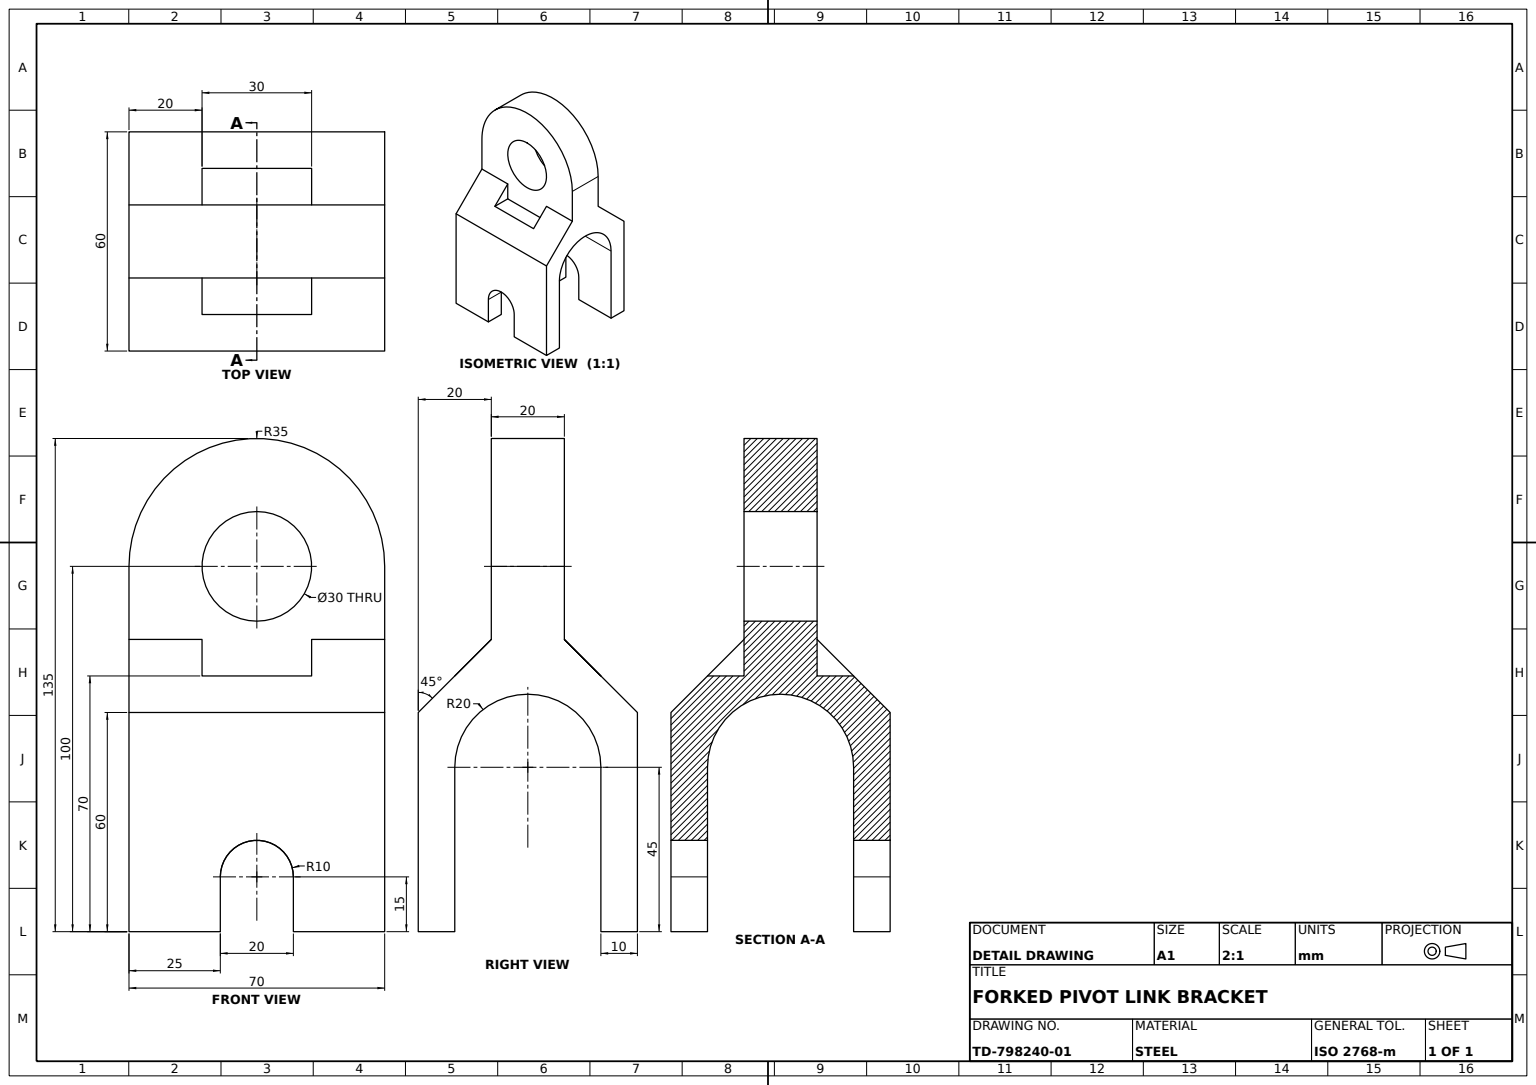
ISO-10303-21;
HEADER;
FILE_DESCRIPTION((''),'2;1');
FILE_NAME('','',(''),(''),'','','');
FILE_SCHEMA(('AUTOMOTIVE_DESIGN'));
ENDSEC;
DATA;
#1=APPLICATION_CONTEXT('');
#2=PRODUCT_CONTEXT('',#1,'mechanical');
#3=PRODUCT('','','',(#2));
#4=PRODUCT_DEFINITION_FORMATION('','',#3);
#5=PRODUCT_DEFINITION_CONTEXT('',#1,'design');
#6=PRODUCT_DEFINITION('','',#4,#5);
#7=PRODUCT_DEFINITION_SHAPE('','',#6);
#8=(LENGTH_UNIT()NAMED_UNIT(*)SI_UNIT(.MILLI.,.METRE.));
#9=(NAMED_UNIT(*)PLANE_ANGLE_UNIT()SI_UNIT($,.RADIAN.));
#10=(NAMED_UNIT(*)SI_UNIT($,.STERADIAN.)SOLID_ANGLE_UNIT());
#11=UNCERTAINTY_MEASURE_WITH_UNIT(LENGTH_MEASURE(0.005),#8,'distance_accuracy_value','');
#12=(GEOMETRIC_REPRESENTATION_CONTEXT(3)GLOBAL_UNCERTAINTY_ASSIGNED_CONTEXT((#11))GLOBAL_UNIT_ASSIGNED_CONTEXT((#8,#9,#10))REPRESENTATION_CONTEXT('',''));
#13=CARTESIAN_POINT('',(30.,10.,-15.));
#14=VERTEX_POINT('',#13);
#15=CARTESIAN_POINT('',(30.,-10.,-15.));
#16=VERTEX_POINT('',#15);
#17=CARTESIAN_POINT('',(30.,0.,-15.));
#18=DIRECTION('',(-1.,0.,0.));
#19=DIRECTION('',(0.,0.,1.));
#20=AXIS2_PLACEMENT_3D('',#17,#18,#19);
#21=CIRCLE('',#20,10.);
#22=EDGE_CURVE('',#14,#16,#21,.F.);
#23=ORIENTED_EDGE('',*,*,#22,.T.);
#24=CARTESIAN_POINT('',(20.,-10.,-15.));
#25=VERTEX_POINT('',#24);
#26=CARTESIAN_POINT('',(43.,-10.,-15.));
#27=VECTOR('',#18,1000.);
#28=LINE('',#26,#27);
#29=EDGE_CURVE('',#25,#16,#28,.F.);
#30=ORIENTED_EDGE('',*,*,#29,.F.);
#31=CARTESIAN_POINT('',(20.,10.,-15.));
#32=VERTEX_POINT('',#31);
#33=CARTESIAN_POINT('',(20.,0.,-15.));
#34=AXIS2_PLACEMENT_3D('',#33,#18,#19);
#35=CIRCLE('',#34,10.);
#36=EDGE_CURVE('',#25,#32,#35,.T.);
#37=ORIENTED_EDGE('',*,*,#36,.T.);
#38=CARTESIAN_POINT('',(43.,10.,-15.));
#39=LINE('',#38,#27);
#40=EDGE_CURVE('',#32,#14,#39,.F.);
#41=ORIENTED_EDGE('',*,*,#40,.T.);
#42=EDGE_LOOP('',(#23,#30,#37,#41));
#43=FACE_BOUND('',#42,.T.);
#44=CARTESIAN_POINT('',(43.,0.,-15.));
#45=AXIS2_PLACEMENT_3D('',#44,#18,#19);
#46=CYLINDRICAL_SURFACE('',#45,10.);
#47=ADVANCED_FACE('',(#43),#46,.F.);
#48=CARTESIAN_POINT('',(30.,35.,30.));
#49=VERTEX_POINT('',#48);
#50=CARTESIAN_POINT('',(10.,35.,50.));
#51=VERTEX_POINT('',#50);
#52=DIRECTION('',(-0.707106781,0.,0.707106781));
#53=VECTOR('',#52,1000.);
#54=LINE('',#48,#53);
#55=EDGE_CURVE('',#49,#51,#54,.T.);
#56=ORIENTED_EDGE('',*,*,#55,.F.);
#57=CARTESIAN_POINT('',(30.,35.,-30.));
#58=VERTEX_POINT('',#57);
#59=DIRECTION('',(0.,0.,-1.));
#60=VECTOR('',#59,1000.);
#61=LINE('',#48,#60);
#62=EDGE_CURVE('',#49,#58,#61,.T.);
#63=ORIENTED_EDGE('',*,*,#62,.T.);
#64=CARTESIAN_POINT('',(20.,35.,-30.));
#65=VERTEX_POINT('',#64);
#66=LINE('',#57,#27);
#67=EDGE_CURVE('',#58,#65,#66,.T.);
#68=ORIENTED_EDGE('',*,*,#67,.T.);
#69=CARTESIAN_POINT('',(20.,35.,15.));
#70=VERTEX_POINT('',#69);
#71=CARTESIAN_POINT('',(20.,35.,30.));
#72=VECTOR('',#19,1000.);
#73=LINE('',#71,#72);
#74=EDGE_CURVE('',#65,#70,#73,.T.);
#75=ORIENTED_EDGE('',*,*,#74,.T.);
#76=CARTESIAN_POINT('',(-20.,35.,15.));
#77=VERTEX_POINT('',#76);
#78=CARTESIAN_POINT('',(0.,35.,15.));
#79=DIRECTION('',(0.,1.,0.));
#80=AXIS2_PLACEMENT_3D('',#78,#79,#19);
#81=CIRCLE('',#80,20.);
#82=EDGE_CURVE('',#70,#77,#81,.F.);
#83=ORIENTED_EDGE('',*,*,#82,.T.);
#84=CARTESIAN_POINT('',(-20.,35.,-30.));
#85=VERTEX_POINT('',#84);
#86=CARTESIAN_POINT('',(-20.,35.,30.));
#87=LINE('',#86,#60);
#88=EDGE_CURVE('',#77,#85,#87,.T.);
#89=ORIENTED_EDGE('',*,*,#88,.T.);
#90=CARTESIAN_POINT('',(-30.,35.,-30.));
#91=VERTEX_POINT('',#90);
#92=EDGE_CURVE('',#85,#91,#66,.T.);
#93=ORIENTED_EDGE('',*,*,#92,.T.);
#94=CARTESIAN_POINT('',(-30.,35.,30.));
#95=VERTEX_POINT('',#94);
#96=LINE('',#94,#60);
#97=EDGE_CURVE('',#95,#91,#96,.T.);
#98=ORIENTED_EDGE('',*,*,#97,.F.);
#99=CARTESIAN_POINT('',(-10.,35.,50.));
#100=VERTEX_POINT('',#99);
#101=DIRECTION('',(0.707106781,0.,0.707106781));
#102=VECTOR('',#101,1000.);
#103=LINE('',#94,#102);
#104=EDGE_CURVE('',#95,#100,#103,.T.);
#105=ORIENTED_EDGE('',*,*,#104,.T.);
#106=CARTESIAN_POINT('',(-10.,35.,70.));
#107=VERTEX_POINT('',#106);
#108=CARTESIAN_POINT('',(-10.,35.,19.));
#109=LINE('',#108,#72);
#110=EDGE_CURVE('',#100,#107,#109,.T.);
#111=ORIENTED_EDGE('',*,*,#110,.T.);
#112=CARTESIAN_POINT('',(10.,35.,70.));
#113=VERTEX_POINT('',#112);
#114=LINE('',#112,#27);
#115=EDGE_CURVE('',#113,#107,#114,.T.);
#116=ORIENTED_EDGE('',*,*,#115,.F.);
#117=CARTESIAN_POINT('',(10.,35.,19.));
#118=LINE('',#117,#72);
#119=EDGE_CURVE('',#51,#113,#118,.T.);
#120=ORIENTED_EDGE('',*,*,#119,.F.);
#121=EDGE_LOOP('',(#56,#63,#68,#75,#83,#89,#93,#98,#105,#111,#116,#120));
#122=FACE_BOUND('',#121,.T.);
#123=AXIS2_PLACEMENT_3D('',#48,#79,#19);
#124=PLANE('',#123);
#125=ADVANCED_FACE('',(#122),#124,.T.);
#126=ORIENTED_EDGE('',*,*,#92,.F.);
#127=CARTESIAN_POINT('',(-20.,10.,-30.));
#128=VERTEX_POINT('',#127);
#129=DIRECTION('',(0.,-1.,0.));
#130=VECTOR('',#129,1000.);
#131=LINE('',#84,#130);
#132=EDGE_CURVE('',#85,#128,#131,.T.);
#133=ORIENTED_EDGE('',*,*,#132,.T.);
#134=CARTESIAN_POINT('',(-30.,10.,-30.));
#135=VERTEX_POINT('',#134);
#136=CARTESIAN_POINT('',(30.,10.,-30.));
#137=LINE('',#136,#27);
#138=EDGE_CURVE('',#128,#135,#137,.T.);
#139=ORIENTED_EDGE('',*,*,#138,.T.);
#140=LINE('',#90,#130);
#141=EDGE_CURVE('',#91,#135,#140,.T.);
#142=ORIENTED_EDGE('',*,*,#141,.F.);
#143=EDGE_LOOP('',(#126,#133,#139,#142));
#144=FACE_BOUND('',#143,.T.);
#145=AXIS2_PLACEMENT_3D('',#57,#59,#18);
#146=PLANE('',#145);
#147=ADVANCED_FACE('',(#144),#146,.T.);
#148=ORIENTED_EDGE('',*,*,#88,.F.);
#149=CARTESIAN_POINT('',(-20.,-35.,15.));
#150=VERTEX_POINT('',#149);
#151=CARTESIAN_POINT('',(-20.,-50.,15.));
#152=VECTOR('',#79,1000.);
#153=LINE('',#151,#152);
#154=EDGE_CURVE('',#77,#150,#153,.F.);
#155=ORIENTED_EDGE('',*,*,#154,.T.);
#156=CARTESIAN_POINT('',(-20.,-35.,-30.));
#157=VERTEX_POINT('',#156);
#158=LINE('',#156,#72);
#159=EDGE_CURVE('',#157,#150,#158,.T.);
#160=ORIENTED_EDGE('',*,*,#159,.F.);
#161=CARTESIAN_POINT('',(-20.,-10.,-30.));
#162=VERTEX_POINT('',#161);
#163=EDGE_CURVE('',#162,#157,#131,.T.);
#164=ORIENTED_EDGE('',*,*,#163,.F.);
#165=CARTESIAN_POINT('',(-20.,-10.,-15.));
#166=VERTEX_POINT('',#165);
#167=LINE('',#165,#60);
#168=EDGE_CURVE('',#166,#162,#167,.T.);
#169=ORIENTED_EDGE('',*,*,#168,.F.);
#170=CARTESIAN_POINT('',(-20.,10.,-15.));
#171=VERTEX_POINT('',#170);
#172=CARTESIAN_POINT('',(-20.,0.,-15.));
#173=DIRECTION('',(1.,0.,0.));
#174=AXIS2_PLACEMENT_3D('',#172,#173,#59);
#175=CIRCLE('',#174,10.);
#176=EDGE_CURVE('',#171,#166,#175,.T.);
#177=ORIENTED_EDGE('',*,*,#176,.F.);
#178=CARTESIAN_POINT('',(-20.,10.,-35.));
#179=LINE('',#178,#72);
#180=EDGE_CURVE('',#128,#171,#179,.T.);
#181=ORIENTED_EDGE('',*,*,#180,.F.);
#182=ORIENTED_EDGE('',*,*,#132,.F.);
#183=EDGE_LOOP('',(#148,#155,#160,#164,#169,#177,#181,#182));
#184=FACE_BOUND('',#183,.T.);
#185=AXIS2_PLACEMENT_3D('',#151,#173,#59);
#186=PLANE('',#185);
#187=ADVANCED_FACE('',(#184),#186,.T.);
#188=CARTESIAN_POINT('',(-10.,15.,50.));
#189=VERTEX_POINT('',#188);
#190=CARTESIAN_POINT('',(-10.,-35.,50.));
#191=LINE('',#190,#152);
#192=EDGE_CURVE('',#189,#100,#191,.T.);
#193=ORIENTED_EDGE('',*,*,#192,.T.);
#194=ORIENTED_EDGE('',*,*,#104,.F.);
#195=CARTESIAN_POINT('',(-30.,-35.,30.));
#196=VERTEX_POINT('',#195);
#197=LINE('',#195,#152);
#198=EDGE_CURVE('',#196,#95,#197,.T.);
#199=ORIENTED_EDGE('',*,*,#198,.F.);
#200=VERTEX_POINT('',#190);
#201=LINE('',#195,#102);
#202=EDGE_CURVE('',#196,#200,#201,.T.);
#203=ORIENTED_EDGE('',*,*,#202,.T.);
#204=CARTESIAN_POINT('',(-10.,-15.,50.));
#205=VERTEX_POINT('',#204);
#206=EDGE_CURVE('',#200,#205,#191,.T.);
#207=ORIENTED_EDGE('',*,*,#206,.T.);
#208=CARTESIAN_POINT('',(-20.,-15.,40.));
#209=VERTEX_POINT('',#208);
#210=CARTESIAN_POINT('',(-30.,-15.,30.));
#211=DIRECTION('',(-0.707106781,0.,-0.707106781));
#212=VECTOR('',#211,1000.);
#213=LINE('',#210,#212);
#214=EDGE_CURVE('',#205,#209,#213,.T.);
#215=ORIENTED_EDGE('',*,*,#214,.T.);
#216=CARTESIAN_POINT('',(-20.,15.,40.));
#217=VERTEX_POINT('',#216);
#218=LINE('',#216,#130);
#219=EDGE_CURVE('',#217,#209,#218,.T.);
#220=ORIENTED_EDGE('',*,*,#219,.F.);
#221=CARTESIAN_POINT('',(-30.,15.,30.));
#222=LINE('',#221,#102);
#223=EDGE_CURVE('',#217,#189,#222,.T.);
#224=ORIENTED_EDGE('',*,*,#223,.T.);
#225=EDGE_LOOP('',(#193,#194,#199,#203,#207,#215,#220,#224));
#226=FACE_BOUND('',#225,.T.);
#227=AXIS2_PLACEMENT_3D('',#195,#52,#101);
#228=PLANE('',#227);
#229=ADVANCED_FACE('',(#226),#228,.T.);
#230=ORIENTED_EDGE('',*,*,#141,.T.);
#231=CARTESIAN_POINT('',(-30.,10.,-15.));
#232=VERTEX_POINT('',#231);
#233=CARTESIAN_POINT('',(-30.,10.,0.));
#234=LINE('',#233,#72);
#235=EDGE_CURVE('',#135,#232,#234,.T.);
#236=ORIENTED_EDGE('',*,*,#235,.T.);
#237=CARTESIAN_POINT('',(-30.,-10.,-15.));
#238=VERTEX_POINT('',#237);
#239=CARTESIAN_POINT('',(-30.,0.,-15.));
#240=AXIS2_PLACEMENT_3D('',#239,#18,#19);
#241=CIRCLE('',#240,10.);
#242=EDGE_CURVE('',#232,#238,#241,.F.);
#243=ORIENTED_EDGE('',*,*,#242,.T.);
#244=CARTESIAN_POINT('',(-30.,-10.,-30.));
#245=VERTEX_POINT('',#244);
#246=CARTESIAN_POINT('',(-30.,-10.,0.));
#247=LINE('',#246,#60);
#248=EDGE_CURVE('',#238,#245,#247,.T.);
#249=ORIENTED_EDGE('',*,*,#248,.T.);
#250=CARTESIAN_POINT('',(-30.,-35.,-30.));
#251=VERTEX_POINT('',#250);
#252=EDGE_CURVE('',#245,#251,#140,.T.);
#253=ORIENTED_EDGE('',*,*,#252,.T.);
#254=LINE('',#250,#72);
#255=EDGE_CURVE('',#251,#196,#254,.T.);
#256=ORIENTED_EDGE('',*,*,#255,.T.);
#257=ORIENTED_EDGE('',*,*,#198,.T.);
#258=ORIENTED_EDGE('',*,*,#97,.T.);
#259=EDGE_LOOP('',(#230,#236,#243,#249,#253,#256,#257,#258));
#260=FACE_BOUND('',#259,.T.);
#261=CARTESIAN_POINT('',(-30.,0.,0.));
#262=AXIS2_PLACEMENT_3D('',#261,#18,#19);
#263=PLANE('',#262);
#264=ADVANCED_FACE('',(#260),#263,.T.);
#265=CARTESIAN_POINT('',(10.,0.,85.));
#266=VERTEX_POINT('',#265);
#267=CARTESIAN_POINT('',(10.,0.,70.));
#268=AXIS2_PLACEMENT_3D('',#267,#18,#19);
#269=CIRCLE('',#268,15.);
#270=EDGE_CURVE('',#266,#266,#269,.T.);
#271=ORIENTED_EDGE('',*,*,#270,.F.);
#272=EDGE_LOOP('',(#271));
#273=FACE_BOUND('',#272,.T.);
#274=CARTESIAN_POINT('',(-10.,0.,55.));
#275=VERTEX_POINT('',#274);
#276=CARTESIAN_POINT('',(-10.,0.,70.));
#277=AXIS2_PLACEMENT_3D('',#276,#173,#59);
#278=CIRCLE('',#277,15.);
#279=EDGE_CURVE('',#275,#275,#278,.T.);
#280=ORIENTED_EDGE('',*,*,#279,.F.);
#281=EDGE_LOOP('',(#280));
#282=FACE_BOUND('',#281,.T.);
#283=CYLINDRICAL_SURFACE('',#268,15.);
#284=ADVANCED_FACE('',(#273,#282),#283,.F.);
#285=CARTESIAN_POINT('',(10.,-35.,50.));
#286=VERTEX_POINT('',#285);
#287=CARTESIAN_POINT('',(10.,-15.,50.));
#288=VERTEX_POINT('',#287);
#289=LINE('',#285,#152);
#290=EDGE_CURVE('',#286,#288,#289,.T.);
#291=ORIENTED_EDGE('',*,*,#290,.F.);
#292=CARTESIAN_POINT('',(30.,-35.,30.));
#293=VERTEX_POINT('',#292);
#294=LINE('',#292,#53);
#295=EDGE_CURVE('',#293,#286,#294,.T.);
#296=ORIENTED_EDGE('',*,*,#295,.F.);
#297=LINE('',#292,#152);
#298=EDGE_CURVE('',#293,#49,#297,.T.);
#299=ORIENTED_EDGE('',*,*,#298,.T.);
#300=ORIENTED_EDGE('',*,*,#55,.T.);
#301=CARTESIAN_POINT('',(10.,15.,50.));
#302=VERTEX_POINT('',#301);
#303=EDGE_CURVE('',#302,#51,#289,.T.);
#304=ORIENTED_EDGE('',*,*,#303,.F.);
#305=CARTESIAN_POINT('',(20.,15.,40.));
#306=VERTEX_POINT('',#305);
#307=CARTESIAN_POINT('',(30.,15.,30.));
#308=DIRECTION('',(0.707106781,0.,-0.707106781));
#309=VECTOR('',#308,1000.);
#310=LINE('',#307,#309);
#311=EDGE_CURVE('',#302,#306,#310,.T.);
#312=ORIENTED_EDGE('',*,*,#311,.T.);
#313=CARTESIAN_POINT('',(20.,-15.,40.));
#314=VERTEX_POINT('',#313);
#315=LINE('',#305,#130);
#316=EDGE_CURVE('',#306,#314,#315,.T.);
#317=ORIENTED_EDGE('',*,*,#316,.T.);
#318=CARTESIAN_POINT('',(30.,-15.,30.));
#319=LINE('',#318,#53);
#320=EDGE_CURVE('',#314,#288,#319,.T.);
#321=ORIENTED_EDGE('',*,*,#320,.T.);
#322=EDGE_LOOP('',(#291,#296,#299,#300,#304,#312,#317,#321));
#323=FACE_BOUND('',#322,.T.);
#324=AXIS2_PLACEMENT_3D('',#292,#211,#52);
#325=PLANE('',#324);
#326=ADVANCED_FACE('',(#323),#325,.F.);
#327=VERTEX_POINT('',#136);
#328=CARTESIAN_POINT('',(20.,10.,-30.));
#329=VERTEX_POINT('',#328);
#330=EDGE_CURVE('',#327,#329,#137,.T.);
#331=ORIENTED_EDGE('',*,*,#330,.F.);
#332=CARTESIAN_POINT('',(30.,10.,0.));
#333=LINE('',#332,#72);
#334=EDGE_CURVE('',#327,#14,#333,.T.);
#335=ORIENTED_EDGE('',*,*,#334,.T.);
#336=ORIENTED_EDGE('',*,*,#40,.F.);
#337=CARTESIAN_POINT('',(20.,10.,-35.));
#338=LINE('',#337,#60);
#339=EDGE_CURVE('',#32,#329,#338,.T.);
#340=ORIENTED_EDGE('',*,*,#339,.T.);
#341=EDGE_LOOP('',(#331,#335,#336,#340));
#342=FACE_BOUND('',#341,.T.);
#343=CARTESIAN_POINT('',(43.,10.,-35.));
#344=AXIS2_PLACEMENT_3D('',#343,#129,#59);
#345=PLANE('',#344);
#346=ADVANCED_FACE('',(#342),#345,.T.);
#347=CARTESIAN_POINT('',(10.,-15.,40.));
#348=VERTEX_POINT('',#347);
#349=LINE('',#313,#27);
#350=EDGE_CURVE('',#348,#314,#349,.F.);
#351=ORIENTED_EDGE('',*,*,#350,.T.);
#352=ORIENTED_EDGE('',*,*,#316,.F.);
#353=CARTESIAN_POINT('',(10.,15.,40.));
#354=VERTEX_POINT('',#353);
#355=VECTOR('',#173,1000.);
#356=LINE('',#353,#355);
#357=EDGE_CURVE('',#306,#354,#356,.F.);
#358=ORIENTED_EDGE('',*,*,#357,.T.);
#359=LINE('',#347,#152);
#360=EDGE_CURVE('',#348,#354,#359,.T.);
#361=ORIENTED_EDGE('',*,*,#360,.F.);
#362=EDGE_LOOP('',(#351,#352,#358,#361));
#363=FACE_BOUND('',#362,.T.);
#364=CARTESIAN_POINT('',(0.,0.,40.));
#365=AXIS2_PLACEMENT_3D('',#364,#59,#18);
#366=PLANE('',#365);
#367=ADVANCED_FACE('',(#363),#366,.F.);
#368=CARTESIAN_POINT('',(30.,-35.,-30.));
#369=VERTEX_POINT('',#368);
#370=CARTESIAN_POINT('',(20.,-35.,-30.));
#371=VERTEX_POINT('',#370);
#372=LINE('',#368,#27);
#373=EDGE_CURVE('',#369,#371,#372,.T.);
#374=ORIENTED_EDGE('',*,*,#373,.F.);
#375=LINE('',#368,#72);
#376=EDGE_CURVE('',#369,#293,#375,.T.);
#377=ORIENTED_EDGE('',*,*,#376,.T.);
#378=ORIENTED_EDGE('',*,*,#295,.T.);
#379=CARTESIAN_POINT('',(10.,-35.,70.));
#380=VERTEX_POINT('',#379);
#381=LINE('',#379,#60);
#382=EDGE_CURVE('',#380,#286,#381,.T.);
#383=ORIENTED_EDGE('',*,*,#382,.F.);
#384=CARTESIAN_POINT('',(-10.,-35.,70.));
#385=VERTEX_POINT('',#384);
#386=LINE('',#379,#27);
#387=EDGE_CURVE('',#380,#385,#386,.T.);
#388=ORIENTED_EDGE('',*,*,#387,.T.);
#389=LINE('',#384,#60);
#390=EDGE_CURVE('',#385,#200,#389,.T.);
#391=ORIENTED_EDGE('',*,*,#390,.T.);
#392=ORIENTED_EDGE('',*,*,#202,.F.);
#393=ORIENTED_EDGE('',*,*,#255,.F.);
#394=EDGE_CURVE('',#157,#251,#372,.T.);
#395=ORIENTED_EDGE('',*,*,#394,.F.);
#396=ORIENTED_EDGE('',*,*,#159,.T.);
#397=CARTESIAN_POINT('',(20.,-35.,15.));
#398=VERTEX_POINT('',#397);
#399=CARTESIAN_POINT('',(0.,-35.,15.));
#400=AXIS2_PLACEMENT_3D('',#399,#129,#59);
#401=CIRCLE('',#400,20.);
#402=EDGE_CURVE('',#150,#398,#401,.F.);
#403=ORIENTED_EDGE('',*,*,#402,.T.);
#404=LINE('',#370,#60);
#405=EDGE_CURVE('',#398,#371,#404,.T.);
#406=ORIENTED_EDGE('',*,*,#405,.T.);
#407=EDGE_LOOP('',(#374,#377,#378,#383,#388,#391,#392,#393,#395,#396,#403,#406));
#408=FACE_BOUND('',#407,.T.);
#409=AXIS2_PLACEMENT_3D('',#368,#129,#59);
#410=PLANE('',#409);
#411=ADVANCED_FACE('',(#408),#410,.T.);
#412=AXIS2_PLACEMENT_3D('',#267,#173,#79);
#413=CIRCLE('',#412,35.);
#414=EDGE_CURVE('',#113,#380,#413,.T.);
#415=ORIENTED_EDGE('',*,*,#414,.F.);
#416=ORIENTED_EDGE('',*,*,#115,.T.);
#417=AXIS2_PLACEMENT_3D('',#276,#173,#79);
#418=CIRCLE('',#417,35.);
#419=EDGE_CURVE('',#107,#385,#418,.T.);
#420=ORIENTED_EDGE('',*,*,#419,.T.);
#421=ORIENTED_EDGE('',*,*,#387,.F.);
#422=EDGE_LOOP('',(#415,#416,#420,#421));
#423=FACE_BOUND('',#422,.T.);
#424=CYLINDRICAL_SURFACE('',#268,35.);
#425=ADVANCED_FACE('',(#423),#424,.T.);
#426=CARTESIAN_POINT('',(-10.,-15.,40.));
#427=VERTEX_POINT('',#426);
#428=LINE('',#208,#355);
#429=EDGE_CURVE('',#427,#209,#428,.F.);
#430=ORIENTED_EDGE('',*,*,#429,.F.);
#431=CARTESIAN_POINT('',(-10.,15.,40.));
#432=VERTEX_POINT('',#431);
#433=LINE('',#426,#152);
#434=EDGE_CURVE('',#427,#432,#433,.T.);
#435=ORIENTED_EDGE('',*,*,#434,.T.);
#436=LINE('',#431,#27);
#437=EDGE_CURVE('',#217,#432,#436,.F.);
#438=ORIENTED_EDGE('',*,*,#437,.F.);
#439=ORIENTED_EDGE('',*,*,#219,.T.);
#440=EDGE_LOOP('',(#430,#435,#438,#439));
#441=FACE_BOUND('',#440,.T.);
#442=AXIS2_PLACEMENT_3D('',#364,#19,#173);
#443=PLANE('',#442);
#444=ADVANCED_FACE('',(#441),#443,.T.);
#445=ORIENTED_EDGE('',*,*,#110,.F.);
#446=ORIENTED_EDGE('',*,*,#192,.F.);
#447=CARTESIAN_POINT('',(-10.,15.,58.5));
#448=LINE('',#447,#60);
#449=EDGE_CURVE('',#189,#432,#448,.T.);
#450=ORIENTED_EDGE('',*,*,#449,.T.);
#451=ORIENTED_EDGE('',*,*,#434,.F.);
#452=CARTESIAN_POINT('',(-10.,-15.,58.5));
#453=LINE('',#452,#60);
#454=EDGE_CURVE('',#205,#427,#453,.T.);
#455=ORIENTED_EDGE('',*,*,#454,.F.);
#456=ORIENTED_EDGE('',*,*,#206,.F.);
#457=ORIENTED_EDGE('',*,*,#390,.F.);
#458=ORIENTED_EDGE('',*,*,#419,.F.);
#459=EDGE_LOOP('',(#445,#446,#450,#451,#455,#456,#457,#458));
#460=FACE_BOUND('',#459,.T.);
#461=ORIENTED_EDGE('',*,*,#279,.T.);
#462=EDGE_LOOP('',(#461));
#463=FACE_BOUND('',#462,.T.);
#464=PLANE('',#277);
#465=ADVANCED_FACE('',(#460,#463),#464,.F.);
#466=ORIENTED_EDGE('',*,*,#334,.F.);
#467=LINE('',#57,#130);
#468=EDGE_CURVE('',#58,#327,#467,.T.);
#469=ORIENTED_EDGE('',*,*,#468,.F.);
#470=ORIENTED_EDGE('',*,*,#62,.F.);
#471=ORIENTED_EDGE('',*,*,#298,.F.);
#472=ORIENTED_EDGE('',*,*,#376,.F.);
#473=CARTESIAN_POINT('',(30.,-10.,-30.));
#474=VERTEX_POINT('',#473);
#475=EDGE_CURVE('',#474,#369,#467,.T.);
#476=ORIENTED_EDGE('',*,*,#475,.F.);
#477=CARTESIAN_POINT('',(30.,-10.,0.));
#478=LINE('',#477,#60);
#479=EDGE_CURVE('',#16,#474,#478,.T.);
#480=ORIENTED_EDGE('',*,*,#479,.F.);
#481=ORIENTED_EDGE('',*,*,#22,.F.);
#482=EDGE_LOOP('',(#466,#469,#470,#471,#472,#476,#480,#481));
#483=FACE_BOUND('',#482,.T.);
#484=CARTESIAN_POINT('',(30.,0.,0.));
#485=AXIS2_PLACEMENT_3D('',#484,#18,#19);
#486=PLANE('',#485);
#487=ADVANCED_FACE('',(#483),#486,.F.);
#488=ORIENTED_EDGE('',*,*,#350,.F.);
#489=CARTESIAN_POINT('',(10.,-15.,58.5));
#490=LINE('',#489,#60);
#491=EDGE_CURVE('',#288,#348,#490,.T.);
#492=ORIENTED_EDGE('',*,*,#491,.F.);
#493=ORIENTED_EDGE('',*,*,#320,.F.);
#494=EDGE_LOOP('',(#488,#492,#493));
#495=FACE_BOUND('',#494,.T.);
#496=CARTESIAN_POINT('',(20.,-15.,58.5));
#497=AXIS2_PLACEMENT_3D('',#496,#129,#173);
#498=PLANE('',#497);
#499=ADVANCED_FACE('',(#495),#498,.F.);
#500=ORIENTED_EDGE('',*,*,#394,.T.);
#501=ORIENTED_EDGE('',*,*,#252,.F.);
#502=LINE('',#473,#355);
#503=EDGE_CURVE('',#245,#162,#502,.T.);
#504=ORIENTED_EDGE('',*,*,#503,.T.);
#505=ORIENTED_EDGE('',*,*,#163,.T.);
#506=EDGE_LOOP('',(#500,#501,#504,#505));
#507=FACE_BOUND('',#506,.T.);
#508=ADVANCED_FACE('',(#507),#146,.T.);
#509=EDGE_CURVE('',#232,#171,#39,.F.);
#510=ORIENTED_EDGE('',*,*,#509,.T.);
#511=ORIENTED_EDGE('',*,*,#176,.T.);
#512=EDGE_CURVE('',#238,#166,#28,.F.);
#513=ORIENTED_EDGE('',*,*,#512,.F.);
#514=ORIENTED_EDGE('',*,*,#242,.F.);
#515=EDGE_LOOP('',(#510,#511,#513,#514));
#516=FACE_BOUND('',#515,.T.);
#517=ADVANCED_FACE('',(#516),#46,.F.);
#518=ORIENTED_EDGE('',*,*,#512,.T.);
#519=ORIENTED_EDGE('',*,*,#168,.T.);
#520=ORIENTED_EDGE('',*,*,#503,.F.);
#521=ORIENTED_EDGE('',*,*,#248,.F.);
#522=EDGE_LOOP('',(#518,#519,#520,#521));
#523=FACE_BOUND('',#522,.T.);
#524=AXIS2_PLACEMENT_3D('',#26,#79,#19);
#525=PLANE('',#524);
#526=ADVANCED_FACE('',(#523),#525,.T.);
#527=ORIENTED_EDGE('',*,*,#479,.T.);
#528=CARTESIAN_POINT('',(20.,-10.,-30.));
#529=VERTEX_POINT('',#528);
#530=EDGE_CURVE('',#529,#474,#502,.T.);
#531=ORIENTED_EDGE('',*,*,#530,.F.);
#532=LINE('',#24,#72);
#533=EDGE_CURVE('',#529,#25,#532,.T.);
#534=ORIENTED_EDGE('',*,*,#533,.T.);
#535=ORIENTED_EDGE('',*,*,#29,.T.);
#536=EDGE_LOOP('',(#527,#531,#534,#535));
#537=FACE_BOUND('',#536,.T.);
#538=ADVANCED_FACE('',(#537),#525,.T.);
#539=ORIENTED_EDGE('',*,*,#509,.F.);
#540=ORIENTED_EDGE('',*,*,#235,.F.);
#541=ORIENTED_EDGE('',*,*,#138,.F.);
#542=ORIENTED_EDGE('',*,*,#180,.T.);
#543=EDGE_LOOP('',(#539,#540,#541,#542));
#544=FACE_BOUND('',#543,.T.);
#545=ADVANCED_FACE('',(#544),#345,.T.);
#546=LINE('',#64,#152);
#547=EDGE_CURVE('',#371,#529,#546,.T.);
#548=ORIENTED_EDGE('',*,*,#547,.F.);
#549=ORIENTED_EDGE('',*,*,#405,.F.);
#550=CARTESIAN_POINT('',(20.,-50.,15.));
#551=LINE('',#550,#152);
#552=EDGE_CURVE('',#70,#398,#551,.F.);
#553=ORIENTED_EDGE('',*,*,#552,.F.);
#554=ORIENTED_EDGE('',*,*,#74,.F.);
#555=EDGE_CURVE('',#329,#65,#546,.T.);
#556=ORIENTED_EDGE('',*,*,#555,.F.);
#557=ORIENTED_EDGE('',*,*,#339,.F.);
#558=ORIENTED_EDGE('',*,*,#36,.F.);
#559=ORIENTED_EDGE('',*,*,#533,.F.);
#560=EDGE_LOOP('',(#548,#549,#553,#554,#556,#557,#558,#559));
#561=FACE_BOUND('',#560,.T.);
#562=CARTESIAN_POINT('',(20.,-50.,-45.));
#563=AXIS2_PLACEMENT_3D('',#562,#18,#19);
#564=PLANE('',#563);
#565=ADVANCED_FACE('',(#561),#564,.T.);
#566=ORIENTED_EDGE('',*,*,#429,.T.);
#567=ORIENTED_EDGE('',*,*,#214,.F.);
#568=ORIENTED_EDGE('',*,*,#454,.T.);
#569=EDGE_LOOP('',(#566,#567,#568));
#570=FACE_BOUND('',#569,.T.);
#571=CARTESIAN_POINT('',(-20.,-15.,58.5));
#572=AXIS2_PLACEMENT_3D('',#571,#79,#18);
#573=PLANE('',#572);
#574=ADVANCED_FACE('',(#570),#573,.T.);
#575=ORIENTED_EDGE('',*,*,#475,.T.);
#576=ORIENTED_EDGE('',*,*,#373,.T.);
#577=ORIENTED_EDGE('',*,*,#547,.T.);
#578=ORIENTED_EDGE('',*,*,#530,.T.);
#579=EDGE_LOOP('',(#575,#576,#577,#578));
#580=FACE_BOUND('',#579,.T.);
#581=ADVANCED_FACE('',(#580),#146,.T.);
#582=ORIENTED_EDGE('',*,*,#449,.F.);
#583=ORIENTED_EDGE('',*,*,#223,.F.);
#584=ORIENTED_EDGE('',*,*,#437,.T.);
#585=EDGE_LOOP('',(#582,#583,#584));
#586=FACE_BOUND('',#585,.T.);
#587=AXIS2_PLACEMENT_3D('',#447,#129,#173);
#588=PLANE('',#587);
#589=ADVANCED_FACE('',(#586),#588,.T.);
#590=ORIENTED_EDGE('',*,*,#414,.T.);
#591=ORIENTED_EDGE('',*,*,#382,.T.);
#592=ORIENTED_EDGE('',*,*,#290,.T.);
#593=ORIENTED_EDGE('',*,*,#491,.T.);
#594=ORIENTED_EDGE('',*,*,#360,.T.);
#595=CARTESIAN_POINT('',(10.,15.,58.5));
#596=LINE('',#595,#60);
#597=EDGE_CURVE('',#302,#354,#596,.T.);
#598=ORIENTED_EDGE('',*,*,#597,.F.);
#599=ORIENTED_EDGE('',*,*,#303,.T.);
#600=ORIENTED_EDGE('',*,*,#119,.T.);
#601=EDGE_LOOP('',(#590,#591,#592,#593,#594,#598,#599,#600));
#602=FACE_BOUND('',#601,.T.);
#603=ORIENTED_EDGE('',*,*,#270,.T.);
#604=EDGE_LOOP('',(#603));
#605=FACE_BOUND('',#604,.T.);
#606=AXIS2_PLACEMENT_3D('',#267,#173,#59);
#607=PLANE('',#606);
#608=ADVANCED_FACE('',(#602,#605),#607,.T.);
#609=ORIENTED_EDGE('',*,*,#154,.F.);
#610=ORIENTED_EDGE('',*,*,#82,.F.);
#611=ORIENTED_EDGE('',*,*,#552,.T.);
#612=ORIENTED_EDGE('',*,*,#402,.F.);
#613=EDGE_LOOP('',(#609,#610,#611,#612));
#614=FACE_BOUND('',#613,.T.);
#615=CARTESIAN_POINT('',(0.,-50.,15.));
#616=AXIS2_PLACEMENT_3D('',#615,#79,#19);
#617=CYLINDRICAL_SURFACE('',#616,20.);
#618=ADVANCED_FACE('',(#614),#617,.F.);
#619=ORIENTED_EDGE('',*,*,#311,.F.);
#620=ORIENTED_EDGE('',*,*,#597,.T.);
#621=ORIENTED_EDGE('',*,*,#357,.F.);
#622=EDGE_LOOP('',(#619,#620,#621));
#623=FACE_BOUND('',#622,.T.);
#624=AXIS2_PLACEMENT_3D('',#595,#79,#18);
#625=PLANE('',#624);
#626=ADVANCED_FACE('',(#623),#625,.F.);
#627=ORIENTED_EDGE('',*,*,#555,.T.);
#628=ORIENTED_EDGE('',*,*,#67,.F.);
#629=ORIENTED_EDGE('',*,*,#468,.T.);
#630=ORIENTED_EDGE('',*,*,#330,.T.);
#631=EDGE_LOOP('',(#627,#628,#629,#630));
#632=FACE_BOUND('',#631,.T.);
#633=ADVANCED_FACE('',(#632),#146,.T.);
#634=CLOSED_SHELL('',(#47,#125,#147,#187,#229,#264,#284,#326,#346,#367,#411,#425,#444,#465,#487,#499,#508,#517,#526,#538,#545,#565,#574,#581,#589,#608,#618,#626,#633));
#635=MANIFOLD_SOLID_BREP('',#634);
#636=ADVANCED_BREP_SHAPE_REPRESENTATION('',(#635),#12);
#637=SHAPE_DEFINITION_REPRESENTATION(#7,#636);
ENDSEC;
END-ISO-10303-21;
